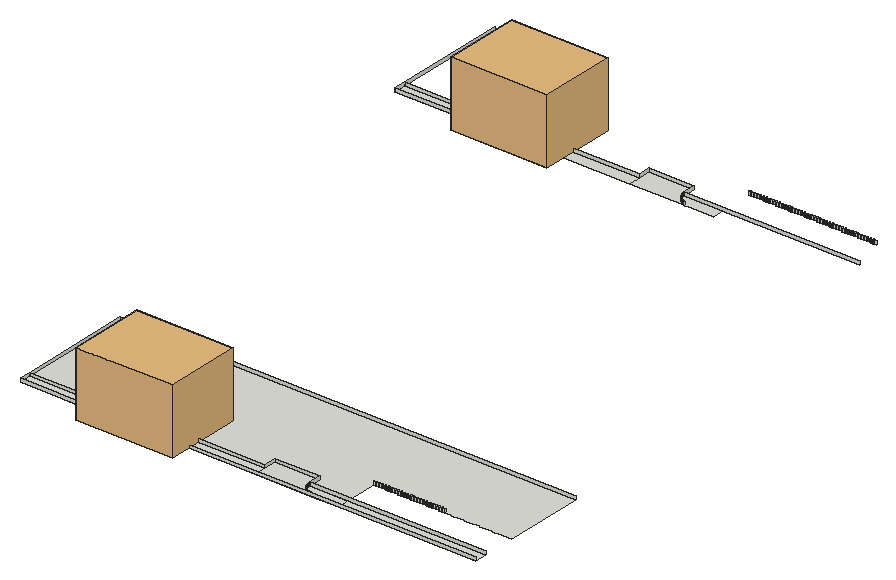
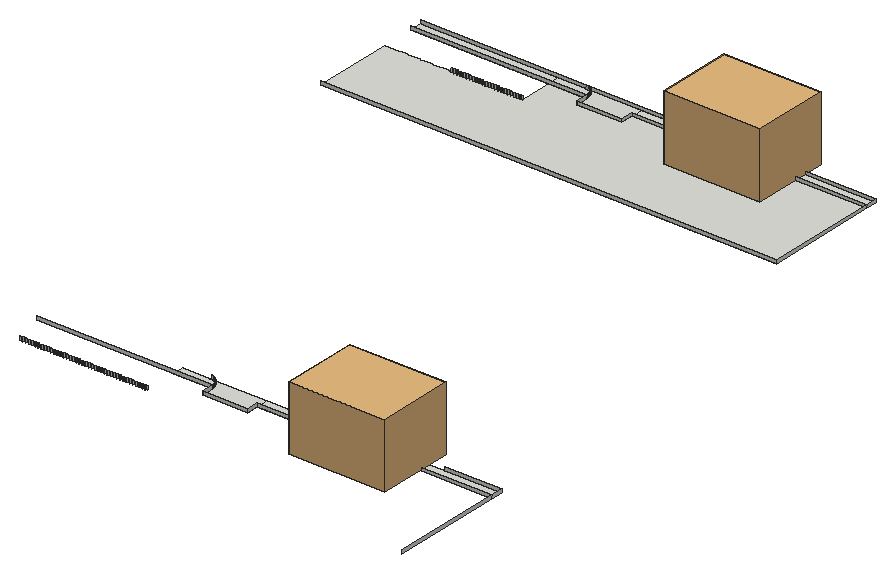
# SketchUp Ruby script. Lengths in inches.
U = 1.inch
M = Sketchup.active_model
def pt(a) = Geom::Point3d.new(a.map { |v| v * U })
def face(e, loops, mat)
  f = e.add_face(loops[0].map { |a| pt(a) })
  loops[1..].each { |l| e.add_face(l.map { |a| pt(a) }).erase! }
  f.material = f.back_material = mat if mat
  f
end
# faces: each face lists its corners as indices into pts; further lists are holes
def faces(e, pts, list, mat = nil) = list.each { |f| face(e, (f[0].is_a?(Array) ? f : [f]).map { |l| l.map { |i| pts[i] } }, mat) }
# xy, xz, yz: faces in a plane at the given z, y or x. An outline is a flat list of corners, or four numbers for a rectangle; further outlines are holes
def ring(l) = l.size == 4 ? [[l[0], l[1]], [l[2], l[1]], [l[2], l[3]], [l[0], l[3]]] : l.each_slice(2).to_a
def flat(e, list, mat, &to3) = list.each { |f| face(e, (f[0].is_a?(Array) ? f : [f]).map { |l| ring(l).map { |u, v| to3.(u, v) } }, mat) }
def xy(e, z, list, mat = nil) = flat(e, list, mat) { |x, y| [x, y, z] }
def xz(e, y, list, mat = nil) = flat(e, list, mat) { |x, z| [x, y, z] }
def yz(e, x, list, mat = nil) = flat(e, list, mat) { |y, z| [x, y, z] }
def lines(e, pts, list) = list.each { |a, b| e.add_line(pt(pts[a]), pt(pts[b])) }
# prism: a flat outline (further loops are holes) pulled along v
def prism(e, loops, v, mat = nil)
  f = face(e, loops, mat); d = Geom::Vector3d.new(v.map { |x| x * U })
  f.pushpull(f.normal.samedirection?(d) ? d.length : -d.length)
end
def box(e, o, s, mat = nil) = prism(e, [[o, [o[0] + s[0], o[1], o[2]], [o[0] + s[0], o[1] + s[1], o[2]], [o[0], o[1] + s[1], o[2]]]], [0, 0, s[2]], mat)
def at(x, y, z, deg = 0) = Geom::Transformation.translation(pt([x, y, z])) * Geom::Transformation.rotation(ORIGIN, Z_AXIS, deg.degrees)
def axes(o, x, y, z) = Geom::Transformation.new([*x, 0, *y, 0, *z, 0, *pt(o).to_a, 1])
def part(name) = M.definitions.add(name)
# library, detail: a bought-in or finely detailed component or shape, given as its bounding box
def library(name, o, s) = part(name).tap { |d| box(d.entities, o, s) }
def detail(e, o, s) = box(e.add_group.entities, o, s)
def put(e, d, t, mat = nil) = e.add_instance(d, t).tap { |i| i.material = mat if mat }
def group(e, t, mat = nil) = e.add_group.tap { |g| g.transformation = t; g.material = mat if mat }.entities
root = M.entities
c1 = library("Sem+nome (1)",[20.77,3.52,-2.22],[96.42,122.82,82.56])
xy(root,-12.3125,[[484.21,147.25,585.4,162.52],[649.69,147.25,651.69,147.38,653.64,147.77,655.53,148.41,657.33,149.3,658.99,150.4,660.49,151.72,661.8,153.22,662.91,154.88,663.8,156.67,664.4375,158.57,664.83,160.52,664.96,162.52,782.4,162.52,782.4,147.25],[782.4,147.25,782.4,178.0625,839.42,178.0625,839.42,162.33,839.55,160.36,839.93,158.43,840.57,156.56,841.4375,154.79,842.53,153.15,843.84,151.67,845.32,150.37,846.96,149.27,848.73,148.4,850.6,147.76,852.53,147.38,854.5,147.25],[854.5,147.25,852.53,147.38,850.6,147.76,848.73,148.4,846.96,149.27,845.32,150.37,843.84,151.67,842.53,153.15,841.4375,154.79,840.57,156.56,839.93,158.43,839.55,160.36,839.42,162.33,888.5,162.33,888.5,147.25],[888.5,147.25,1063.02,162.33],
  [839.42,162.33,839.42,178.0625,782.4,178.0625,782.4,162.52,484.21,162.52,484.21,305.58,1063.02,305.58,1063.02,203.875,1046.875,203.875,1046.875,204.875,1046.125,204.875,1046.125,203.875,1042.875,203.875,1042.875,204.875,1042.125,204.875,1042.125,203.875,1038.875,203.875,1038.875,204.875,1038.125,204.875,1038.125,203.875,1034.875,203.875,1034.875,204.875,1034.125,204.875,1034.125,203.875,1030.875,203.875,1030.875,204.875,1030.125,204.875,1030.125,203.875,1026.875,203.875,1026.875,204.875,1026.125,204.875,1026.125,203.875,1022.875,203.875,1022.875,204.875,1022.125,204.875,1022.125,203.875,1018.875,203.875,1018.875,204.875,1018.125,204.875,1018.125,203.875,1014.875,203.875,1014.875,204.875,1014.125,204.875,1014.125,203.875,1010.875,203.875,1010.875,204.875,1010.125,204.875,1010.125,203.875,1006.875,203.875,1006.875,204.875,1006.125,204.875,1006.125,203.875,1002.875,203.875,1002.875,204.875,1002.125,204.875,1002.125,203.875,998.875,203.875,998.875,204.875,998.125,204.875,998.125,203.875,994.875,203.875,994.875,204.875,994.125,204.875,994.125,203.875,990.875,203.875,990.875,204.875,990.125,204.875,990.125,203.875,986.875,203.875,986.875,204.875,986.125,204.875,986.125,203.875,982.875,203.875,982.875,204.875,982.125,204.875,982.125,203.875,978.875,203.875,978.875,204.875,978.125,204.875,978.125,203.875,974.875,203.875,974.875,204.875,974.125,204.875,974.125,203.875,970.875,203.875,970.875,204.875,970.125,204.875,970.125,203.875,966.875,203.875,966.875,204.875,966.125,204.875,966.125,203.875,962.875,203.875,962.875,204.875,962.125,204.875,962.125,203.875,958.875,203.875,958.875,204.875,958.125,204.875,958.125,203.875,954.875,203.875,954.875,204.875,954.125,204.875,954.125,203.875,950.875,203.875,950.875,204.875,950.125,204.875,950.125,203.875,946.875,203.875,946.875,204.875,946.125,204.875,946.125,203.875,942.875,203.875,942.875,204.875,942.125,204.875,942.125,203.875,938.875,203.875,938.875,204.875,938.125,204.875,938.125,203.875,934.875,203.875,934.875,204.875,934.125,204.875,934.125,203.875,930.875,203.875,930.875,204.875,930.125,204.875,930.125,203.875,926.875,203.875,926.875,204.875,926.125,204.875,926.125,203.875,922.875,203.875,922.875,204.875,922.125,204.875,922.125,203.875,918.875,203.875,918.875,204.875,918.125,204.875,918.125,203.875,914.875,203.875,914.875,204.875,914.125,204.875,914.125,203.875,910.875,203.875,910.875,204.875,910.125,204.875,910.125,203.875,906.875,203.875,906.875,204.875,906.125,204.875,906.125,203.875,902.875,203.875,902.875,204.875,902.125,204.875,902.125,203.875,898.875,203.875,898.875,204.875,898.125,204.875,898.125,203.875,894.875,203.875,894.875,204.875,894.125,204.875,894.125,203.875,890.875,203.875,890.875,204.875,890.125,204.875,890.125,203.875,888.5,203.875,888.5,162.33],[407.52,838.14,508.71,853.41],[573,838.14,575,838.27,576.96,838.66,578.85,839.31,580.64,840.19,582.3,841.3,583.8,842.62,585.12,844.12,586.23,845.78,587.11,847.57,587.75,849.46,588.14,851.42,588.27,853.41,705.71,853.41,705.71,838.14],[705.71,838.14,705.71,868.96,762.73,868.96,762.73,853.22,762.86,851.26,763.24,849.32,763.88,847.45,764.75,845.68,765.85,844.04,767.15,842.5625,768.63,841.26,770.27,840.16,772.04,839.29,773.91,838.66,775.84,838.27,777.8125,838.14],[777.8125,838.14,775.84,838.27,773.91,838.66,772.04,839.29,770.27,840.16,768.63,841.26,767.15,842.5625,765.85,844.04,764.75,845.68,763.88,847.45,763.24,849.32,762.86,851.26,762.73,853.22,811.8125,853.22,811.8125,838.14]])
xz(root,147.25,[[484.21,-12.3125,585.4,-8],[585.4,-12.3125,649.69,-8],[649.69,-12.3125,1063.02,-8]])
xz(root,162.33,[[839.42,-12.3125,1063.02,-8]])
xz(root,162.52,[[484.21,-12.3125,585.4,-8],[585.4,-12.3125,664.96,-8],[664.96,-12.3125,782.4,-8]])
xz(root,178.0625,[[782.4,-12.3125,839.42,-8]])
xz(root,203.875,[[888.5,-12.3125,890.125,-8],[890.875,-12.3125,894.125,-8],[894.875,-12.3125,898.125,-8],[898.875,-12.3125,902.125,-8],[902.875,-12.3125,906.125,-8],
  [906.875,-12.3125,910.125,-8],[910.875,-12.3125,914.125,-8],[914.875,-12.3125,918.125,-8],[918.875,-12.3125,922.125,-8],[922.875,-12.3125,926.125,-8],
  [926.875,-12.3125,930.125,-8],[930.875,-12.3125,934.125,-8],[934.875,-12.3125,938.125,-8],[938.875,-12.3125,942.125,-8],[942.875,-12.3125,946.125,-8],
  [946.875,-12.3125,950.125,-8],[950.875,-12.3125,954.125,-8],[954.875,-12.3125,958.125,-8],[958.875,-12.3125,962.125,-8],[962.875,-12.3125,966.125,-8],
  [966.875,-12.3125,970.125,-8],[970.875,-12.3125,974.125,-8],[974.875,-12.3125,978.125,-8]])
xz(root,204.875,[[890.125,-12.3125,890.875,-8],[894.125,-12.3125,894.875,-8],[898.125,-12.3125,898.875,-8],[902.125,-12.3125,902.875,-8],[906.125,-12.3125,906.875,-8],
  [910.125,-12.3125,910.875,-8],[914.125,-12.3125,914.875,-8],[918.125,-12.3125,918.875,-8],[922.125,-12.3125,922.875,-8],[926.125,-12.3125,926.875,-8],
  [930.125,-12.3125,930.875,-8],[934.125,-12.3125,934.875,-8],[938.125,-12.3125,938.875,-8],[942.125,-12.3125,942.875,-8],[946.125,-12.3125,946.875,-8],
  [950.125,-12.3125,950.875,-8],[954.125,-12.3125,954.875,-8],[958.125,-12.3125,958.875,-8],[962.125,-12.3125,962.875,-8],[966.125,-12.3125,966.875,-8],
  [970.125,-12.3125,970.875,-8],[974.125,-12.3125,974.875,-8]])
xz(root,305.58,[[484.21,-12.3125,1063.02,-8]])
xz(root,838.14,[[407.52,-12.3125,479.21,-8],[508.71,-12.3125,573,-8]])
xz(root,853.22,[[762.73,-12.3125,986.33,-8]])
xz(root,853.41,[[407.52,-12.3125,508.71,-8],[508.71,-12.3125,588.27,-8],[588.27,-12.3125,705.71,-8]])
xz(root,868.96,[[705.71,-12.3125,762.73,-8]])
xz(root,894.77,[[811.8125,-12.3125,813.4375,-8],[814.1875,-12.3125,817.4375,-8],[818.1875,-12.3125,821.4375,-8],[822.1875,-12.3125,825.4375,-8],[826.1875,-12.3125,829.4375,-8],
  [830.1875,-12.3125,833.4375,-8],[834.1875,-12.3125,837.4375,-8],[838.1875,-12.3125,841.4375,-8],[842.1875,-12.3125,845.4375,-8],[846.1875,-12.3125,849.4375,-8],
  [850.1875,-12.3125,853.4375,-8],[854.1875,-12.3125,857.4375,-8],[858.1875,-12.3125,861.4375,-8],[862.1875,-12.3125,865.4375,-8],[866.1875,-12.3125,869.4375,-8],
  [870.1875,-12.3125,873.4375,-8],[874.1875,-12.3125,877.4375,-8],[878.1875,-12.3125,881.4375,-8],[882.1875,-12.3125,885.4375,-8],[886.1875,-12.3125,889.4375,-8],
  [890.1875,-12.3125,893.4375,-8],[894.1875,-12.3125,897.4375,-8],[898.1875,-12.3125,901.4375,-8],[902.1875,-12.3125,905.4375,-8],[906.1875,-12.3125,909.4375,-8],
  [910.1875,-12.3125,913.4375,-8],[914.1875,-12.3125,917.4375,-8],[918.1875,-12.3125,921.4375,-8],[922.1875,-12.3125,925.4375,-8],[926.1875,-12.3125,929.4375,-8],
  [930.1875,-12.3125,933.4375,-8],[934.1875,-12.3125,937.4375,-8],[938.1875,-12.3125,941.4375,-8],[942.1875,-12.3125,945.4375,-8],[946.1875,-12.3125,949.4375,-8],
  [950.1875,-12.3125,953.4375,-8],[954.1875,-12.3125,957.4375,-8],[958.1875,-12.3125,961.4375,-8],[962.1875,-12.3125,965.4375,-8],[966.1875,-12.3125,969.4375,-8],
  [970.1875,-12.3125,973.4375,-8]])
xz(root,895.77,[[813.4375,-12.3125,814.1875,-8],[817.4375,-12.3125,818.1875,-8],[821.4375,-12.3125,822.1875,-8],[825.4375,-12.3125,826.1875,-8],[829.4375,-12.3125,830.1875,-8],
  [833.4375,-12.3125,834.1875,-8],[837.4375,-12.3125,838.1875,-8],[841.4375,-12.3125,842.1875,-8],[845.4375,-12.3125,846.1875,-8],[849.4375,-12.3125,850.1875,-8],
  [853.4375,-12.3125,854.1875,-8],[857.4375,-12.3125,858.1875,-8],[861.4375,-12.3125,862.1875,-8],[865.4375,-12.3125,866.1875,-8],[869.4375,-12.3125,870.1875,-8],
  [873.4375,-12.3125,874.1875,-8],[877.4375,-12.3125,878.1875,-8],[881.4375,-12.3125,882.1875,-8],[885.4375,-12.3125,886.1875,-8],[889.4375,-12.3125,890.1875,-8],
  [893.4375,-12.3125,894.1875,-8],[897.4375,-12.3125,898.1875,-8],[901.4375,-12.3125,902.1875,-8],[905.4375,-12.3125,906.1875,-8],[909.4375,-12.3125,910.1875,-8],
  [913.4375,-12.3125,914.1875,-8],[917.4375,-12.3125,918.1875,-8],[921.4375,-12.3125,922.1875,-8],[925.4375,-12.3125,926.1875,-8],[929.4375,-12.3125,930.1875,-8],
  [933.4375,-12.3125,934.1875,-8],[937.4375,-12.3125,938.1875,-8],[941.4375,-12.3125,942.1875,-8],[945.4375,-12.3125,946.1875,-8],[949.4375,-12.3125,950.1875,-8],
  [953.4375,-12.3125,954.1875,-8],[957.4375,-12.3125,958.1875,-8],[961.4375,-12.3125,962.1875,-8],[965.4375,-12.3125,966.1875,-8],[969.4375,-12.3125,970.1875,-8]])
yz(root,407.52,[[838.14,-12.3125,853.41,-8],[853.41,-12.3125,996.48,-8]])
yz(root,484.21,[[147.25,-12.3125,162.52,-8],[162.52,-12.3125,305.58,-8]])
yz(root,508.71,[[838.14,-12.3125,853.41,-8]])
yz(root,585.4,[[147.25,-12.3125,162.52,-8]])
yz(root,705.71,[[853.41,-12.3125,868.96,-8]])
yz(root,762.73,[[853.22,-12.3125,868.96,-8]])
yz(root,782.4,[[162.52,-12.3125,178.0625,-8]])
yz(root,813.4375,[[894.77,-12.3125,895.77,-8]])
yz(root,814.1875,[[894.77,-12.3125,895.77,-8]])
yz(root,817.4375,[[894.77,-12.3125,895.77,-8]])
yz(root,818.1875,[[894.77,-12.3125,895.77,-8]])
yz(root,821.4375,[[894.77,-12.3125,895.77,-8]])
yz(root,822.1875,[[894.77,-12.3125,895.77,-8]])
yz(root,825.4375,[[894.77,-12.3125,895.77,-8]])
yz(root,826.1875,[[894.77,-12.3125,895.77,-8]])
yz(root,829.4375,[[894.77,-12.3125,895.77,-8]])
yz(root,830.1875,[[894.77,-12.3125,895.77,-8]])
yz(root,833.4375,[[894.77,-12.3125,895.77,-8]])
yz(root,834.1875,[[894.77,-12.3125,895.77,-8]])
yz(root,837.4375,[[894.77,-12.3125,895.77,-8]])
yz(root,838.1875,[[894.77,-12.3125,895.77,-8]])
yz(root,839.42,[[162.33,-12.3125,178.0625,-8]])
yz(root,841.4375,[[894.77,-12.3125,895.77,-8]])
yz(root,842.1875,[[894.77,-12.3125,895.77,-8]])
yz(root,845.4375,[[894.77,-12.3125,895.77,-8]])
yz(root,846.1875,[[894.77,-12.3125,895.77,-8]])
yz(root,849.4375,[[894.77,-12.3125,895.77,-8]])
yz(root,850.1875,[[894.77,-12.3125,895.77,-8]])
yz(root,853.4375,[[894.77,-12.3125,895.77,-8]])
yz(root,854.1875,[[894.77,-12.3125,895.77,-8]])
yz(root,857.4375,[[894.77,-12.3125,895.77,-8]])
yz(root,858.1875,[[894.77,-12.3125,895.77,-8]])
yz(root,861.4375,[[894.77,-12.3125,895.77,-8]])
yz(root,862.1875,[[894.77,-12.3125,895.77,-8]])
yz(root,865.4375,[[894.77,-12.3125,895.77,-8]])
yz(root,866.1875,[[894.77,-12.3125,895.77,-8]])
yz(root,869.4375,[[894.77,-12.3125,895.77,-8]])
yz(root,870.1875,[[894.77,-12.3125,895.77,-8]])
yz(root,873.4375,[[894.77,-12.3125,895.77,-8]])
yz(root,874.1875,[[894.77,-12.3125,895.77,-8]])
yz(root,877.4375,[[894.77,-12.3125,895.77,-8]])
yz(root,878.1875,[[894.77,-12.3125,895.77,-8]])
yz(root,881.4375,[[894.77,-12.3125,895.77,-8]])
yz(root,882.1875,[[894.77,-12.3125,895.77,-8]])
yz(root,885.4375,[[894.77,-12.3125,895.77,-8]])
yz(root,886.1875,[[894.77,-12.3125,895.77,-8]])
yz(root,889.4375,[[894.77,-12.3125,895.77,-8]])
yz(root,890.125,[[203.875,-12.3125,204.875,-8]])
yz(root,890.1875,[[894.77,-12.3125,895.77,-8]])
yz(root,890.875,[[203.875,-12.3125,204.875,-8]])
yz(root,893.4375,[[894.77,-12.3125,895.77,-8]])
yz(root,894.125,[[203.875,-12.3125,204.875,-8]])
yz(root,894.1875,[[894.77,-12.3125,895.77,-8]])
yz(root,894.875,[[203.875,-12.3125,204.875,-8]])
yz(root,897.4375,[[894.77,-12.3125,895.77,-8]])
yz(root,898.125,[[203.875,-12.3125,204.875,-8]])
yz(root,898.1875,[[894.77,-12.3125,895.77,-8]])
yz(root,898.875,[[203.875,-12.3125,204.875,-8]])
yz(root,901.4375,[[894.77,-12.3125,895.77,-8]])
yz(root,902.125,[[203.875,-12.3125,204.875,-8]])
yz(root,902.1875,[[894.77,-12.3125,895.77,-8]])
yz(root,902.875,[[203.875,-12.3125,204.875,-8]])
yz(root,905.4375,[[894.77,-12.3125,895.77,-8]])
yz(root,906.125,[[203.875,-12.3125,204.875,-8]])
yz(root,906.1875,[[894.77,-12.3125,895.77,-8]])
yz(root,906.875,[[203.875,-12.3125,204.875,-8]])
yz(root,909.4375,[[894.77,-12.3125,895.77,-8]])
yz(root,910.125,[[203.875,-12.3125,204.875,-8]])
yz(root,910.1875,[[894.77,-12.3125,895.77,-8]])
yz(root,910.875,[[203.875,-12.3125,204.875,-8]])
yz(root,913.4375,[[894.77,-12.3125,895.77,-8]])
yz(root,914.125,[[203.875,-12.3125,204.875,-8]])
yz(root,914.1875,[[894.77,-12.3125,895.77,-8]])
yz(root,914.875,[[203.875,-12.3125,204.875,-8]])
yz(root,917.4375,[[894.77,-12.3125,895.77,-8]])
yz(root,918.125,[[203.875,-12.3125,204.875,-8]])
yz(root,918.1875,[[894.77,-12.3125,895.77,-8]])
yz(root,918.875,[[203.875,-12.3125,204.875,-8]])
yz(root,921.4375,[[894.77,-12.3125,895.77,-8]])
yz(root,922.125,[[203.875,-12.3125,204.875,-8]])
yz(root,922.1875,[[894.77,-12.3125,895.77,-8]])
yz(root,922.875,[[203.875,-12.3125,204.875,-8]])
yz(root,925.4375,[[894.77,-12.3125,895.77,-8]])
yz(root,926.125,[[203.875,-12.3125,204.875,-8]])
yz(root,926.1875,[[894.77,-12.3125,895.77,-8]])
yz(root,926.875,[[203.875,-12.3125,204.875,-8]])
yz(root,929.4375,[[894.77,-12.3125,895.77,-8]])
yz(root,930.125,[[203.875,-12.3125,204.875,-8]])
yz(root,930.1875,[[894.77,-12.3125,895.77,-8]])
yz(root,930.875,[[203.875,-12.3125,204.875,-8]])
yz(root,933.4375,[[894.77,-12.3125,895.77,-8]])
yz(root,934.125,[[203.875,-12.3125,204.875,-8]])
yz(root,934.1875,[[894.77,-12.3125,895.77,-8]])
yz(root,934.875,[[203.875,-12.3125,204.875,-8]])
yz(root,937.4375,[[894.77,-12.3125,895.77,-8]])
yz(root,938.125,[[203.875,-12.3125,204.875,-8]])
yz(root,938.1875,[[894.77,-12.3125,895.77,-8]])
yz(root,938.875,[[203.875,-12.3125,204.875,-8]])
yz(root,941.4375,[[894.77,-12.3125,895.77,-8]])
yz(root,942.125,[[203.875,-12.3125,204.875,-8]])
yz(root,942.1875,[[894.77,-12.3125,895.77,-8]])
yz(root,942.875,[[203.875,-12.3125,204.875,-8]])
yz(root,945.4375,[[894.77,-12.3125,895.77,-8]])
yz(root,946.125,[[203.875,-12.3125,204.875,-8]])
yz(root,946.1875,[[894.77,-12.3125,895.77,-8]])
yz(root,946.875,[[203.875,-12.3125,204.875,-8]])
yz(root,949.4375,[[894.77,-12.3125,895.77,-8]])
yz(root,950.125,[[203.875,-12.3125,204.875,-8]])
yz(root,950.1875,[[894.77,-12.3125,895.77,-8]])
yz(root,950.875,[[203.875,-12.3125,204.875,-8]])
yz(root,953.4375,[[894.77,-12.3125,895.77,-8]])
yz(root,954.125,[[203.875,-12.3125,204.875,-8]])
yz(root,954.1875,[[894.77,-12.3125,895.77,-8]])
yz(root,954.875,[[203.875,-12.3125,204.875,-8]])
yz(root,957.4375,[[894.77,-12.3125,895.77,-8]])
yz(root,958.125,[[203.875,-12.3125,204.875,-8]])
yz(root,958.1875,[[894.77,-12.3125,895.77,-8]])
yz(root,958.875,[[203.875,-12.3125,204.875,-8]])
yz(root,961.4375,[[894.77,-12.3125,895.77,-8]])
yz(root,962.125,[[203.875,-12.3125,204.875,-8]])
yz(root,962.1875,[[894.77,-12.3125,895.77,-8]])
yz(root,962.875,[[203.875,-12.3125,204.875,-8]])
yz(root,965.4375,[[894.77,-12.3125,895.77,-8]])
yz(root,966.125,[[203.875,-12.3125,204.875,-8]])
yz(root,966.1875,[[894.77,-12.3125,895.77,-8]])
yz(root,966.875,[[203.875,-12.3125,204.875,-8]])
yz(root,969.4375,[[894.77,-12.3125,895.77,-8]])
yz(root,970.125,[[203.875,-12.3125,204.875,-8]])
yz(root,970.1875,[[894.77,-12.3125,895.77,-8]])
yz(root,970.875,[[203.875,-12.3125,204.875,-8]])
yz(root,974.125,[[203.875,-12.3125,204.875,-8]])
yz(root,974.875,[[203.875,-12.3125,204.875,-8]])
yz(root,978.125,[[203.875,-12.3125,204.875,-8]])
p = [[651.69,147.38,-8],[649.69,147.25,-8],[649.69,147.25,-12.3125],[651.69,147.38,-12.3125],[653.64,147.77,-8],[653.64,147.77,-12.3125],
  [852.53,147.38,-8],[850.6,147.76,-8],[850.6,147.76,-12.3125],[852.53,147.38,-12.3125],[655.53,148.41,-8],[655.53,148.41,-12.3125],
  [848.73,148.4,-8],[848.73,148.4,-12.3125],[657.33,149.3,-8],[657.33,149.3,-12.3125],[846.96,149.27,-8],[846.96,149.27,-12.3125],
  [658.99,150.4,-8],[658.99,150.4,-12.3125],[845.32,150.37,-8],[845.32,150.37,-12.3125],[660.49,151.72,-8],[660.49,151.72,-12.3125],
  [843.84,151.67,-8],[843.84,151.67,-12.3125],[661.8,153.22,-8],[661.8,153.22,-12.3125],[842.53,153.15,-8],[842.53,153.15,-12.3125],
  [662.91,154.88,-8],[662.91,154.88,-12.3125],[841.4375,154.79,-8],[841.4375,154.79,-12.3125],[840.57,156.56,-8],[840.57,156.56,-12.3125],
  [663.8,156.67,-8],[663.8,156.67,-12.3125],[839.93,158.43,-8],[839.93,158.43,-12.3125],[664.4375,158.57,-8],[664.4375,158.57,-12.3125],
  [839.55,160.36,-8],[839.55,160.36,-12.3125],[664.83,160.52,-8],[664.83,160.52,-12.3125],[839.42,162.33,-8],[839.42,162.33,-12.3125],
  [664.96,162.52,-8],[664.96,162.52,-12.3125],[575,838.27,-8],[573,838.14,-8],[573,838.14,-12.3125],[575,838.27,-12.3125],
  [576.96,838.66,-8],[576.96,838.66,-12.3125],[775.84,838.27,-8],[773.91,838.66,-8],[773.91,838.66,-12.3125],[775.84,838.27,-12.3125],
  [578.85,839.31,-8],[578.85,839.31,-12.3125],[772.04,839.29,-8],[772.04,839.29,-12.3125],[580.64,840.19,-8],[580.64,840.19,-12.3125],
  [770.27,840.16,-8],[770.27,840.16,-12.3125],[582.3,841.3,-8],[582.3,841.3,-12.3125],[768.63,841.26,-8],[768.63,841.26,-12.3125],
  [583.8,842.62,-8],[583.8,842.62,-12.3125],[767.15,842.5625,-8],[767.15,842.5625,-12.3125],[585.12,844.12,-8],[585.12,844.12,-12.3125],
  [765.85,844.04,-8],[765.85,844.04,-12.3125],[764.75,845.68,-8],[764.75,845.68,-12.3125],[586.23,845.78,-8],[586.23,845.78,-12.3125],
  [763.88,847.45,-8],[763.88,847.45,-12.3125],[587.11,847.57,-8],[587.11,847.57,-12.3125],[763.24,849.32,-8],[763.24,849.32,-12.3125],
  [587.75,849.46,-8],[587.75,849.46,-12.3125],[762.86,851.26,-8],[762.86,851.26,-12.3125],[588.14,851.42,-8],[588.14,851.42,-12.3125],
  [762.73,853.22,-8],[762.73,853.22,-12.3125],[588.27,853.41,-8],[588.27,853.41,-12.3125]]
faces(root,p,[[0,1,2,3],[4,0,3,5],[6,7,8,9],[10,4,5,11],[7,12,13,8],[14,10,11,15],[12,16,17,13],[18,14,15,19],
  [16,20,21,17],[22,18,19,23],[20,24,25,21],[26,22,23,27],[24,28,29,25],[30,26,27,31],[28,32,33,29],[32,34,35,33],
  [36,30,31,37],[34,38,39,35],[40,36,37,41],[38,42,43,39],[44,40,41,45],[42,46,47,43],[48,44,45,49],[50,51,52,53],
  [54,50,53,55],[56,57,58,59],[60,54,55,61],[57,62,63,58],[64,60,61,65],[62,66,67,63],[68,64,65,69],[66,70,71,67],
  [72,68,69,73],[70,74,75,71],[76,72,73,77],[74,78,79,75],[78,80,81,79],[82,76,77,83],[80,84,85,81],[86,82,83,87],
  [84,88,89,85],[90,86,87,91],[88,92,93,89],[94,90,91,95],[92,96,97,93],[98,94,95,99]])
put(root,c1,at(494.79,929.97,-10.09,-90))
put(root,c1,at(571.48,239.07,-10.09,-90))
